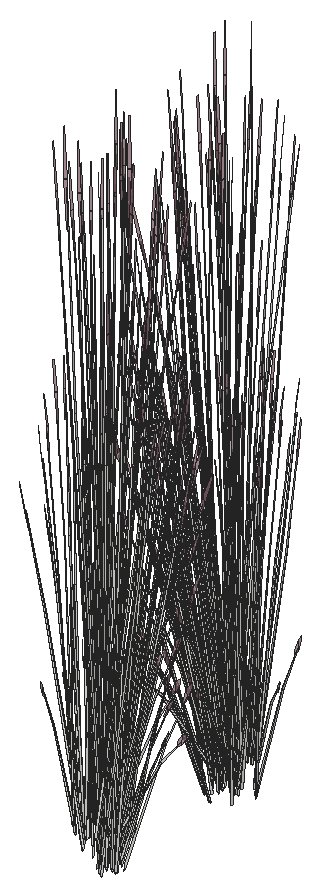
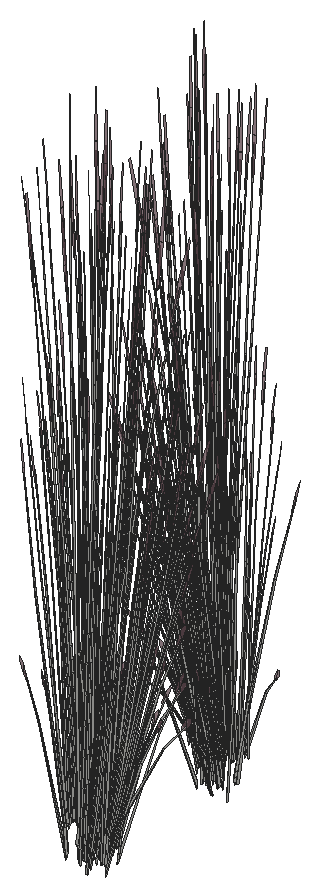
# SketchUp Ruby script. Lengths in inches.
U = 1.inch
M = Sketchup.active_model
def pt(a) = Geom::Point3d.new(a.map { |v| v * U })
def face(e, loops, mat)
  f = e.add_face(loops[0].map { |a| pt(a) })
  loops[1..].each { |l| e.add_face(l.map { |a| pt(a) }).erase! }
  f.material = f.back_material = mat if mat
  f
end
# faces: each face lists its corners as indices into pts; further lists are holes
def faces(e, pts, list, mat = nil) = list.each { |f| face(e, (f[0].is_a?(Array) ? f : [f]).map { |l| l.map { |i| pts[i] } }, mat) }
# xy, xz, yz: faces in a plane at the given z, y or x. An outline is a flat list of corners, or four numbers for a rectangle; further outlines are holes
def ring(l) = l.size == 4 ? [[l[0], l[1]], [l[2], l[1]], [l[2], l[3]], [l[0], l[3]]] : l.each_slice(2).to_a
def flat(e, list, mat, &to3) = list.each { |f| face(e, (f[0].is_a?(Array) ? f : [f]).map { |l| ring(l).map { |u, v| to3.(u, v) } }, mat) }
def xy(e, z, list, mat = nil) = flat(e, list, mat) { |x, y| [x, y, z] }
def xz(e, y, list, mat = nil) = flat(e, list, mat) { |x, z| [x, y, z] }
def yz(e, x, list, mat = nil) = flat(e, list, mat) { |y, z| [x, y, z] }
def lines(e, pts, list) = list.each { |a, b| e.add_line(pt(pts[a]), pt(pts[b])) }
# prism: a flat outline (further loops are holes) pulled along v
def prism(e, loops, v, mat = nil)
  f = face(e, loops, mat); d = Geom::Vector3d.new(v.map { |x| x * U })
  f.pushpull(f.normal.samedirection?(d) ? d.length : -d.length)
end
def box(e, o, s, mat = nil) = prism(e, [[o, [o[0] + s[0], o[1], o[2]], [o[0] + s[0], o[1] + s[1], o[2]], [o[0], o[1] + s[1], o[2]]]], [0, 0, s[2]], mat)
def at(x, y, z, deg = 0) = Geom::Transformation.translation(pt([x, y, z])) * Geom::Transformation.rotation(ORIGIN, Z_AXIS, deg.degrees)
def axes(o, x, y, z) = Geom::Transformation.new([*x, 0, *y, 0, *z, 0, *pt(o).to_a, 1])
def part(name) = M.definitions.add(name)
# library, detail: a bought-in or finely detailed component or shape, given as its bounding box
def library(name, o, s) = part(name).tap { |d| box(d.entities, o, s) }
def detail(e, o, s) = box(e.add_group.entities, o, s)
def put(e, d, t, mat = nil) = e.add_instance(d, t).tap { |i| i.material = mat if mat }
def group(e, t, mat = nil) = e.add_group.tap { |g| g.transformation = t; g.material = mat if mat }.entities
root = M.entities
M.materials.add("LightPink_Translucent").color = [144, 107, 117]
M.materials["LightPink_Translucent"].alpha = 0.75
c1 = part("blade")
p = [[2.15,0.21,22],[0,0.17,0],[0.09,0.45,0],[2.18,0.31,22],[2.29,0.31,22],[0.38,0.45,0],
  [2.48,0.24,33],[2.49,0.24,33],[2.48,0.22,33]]
faces(c1.entities,p,[[0,1,2,3],[4,5,2,3],[6,3,4,7],[8,0,3,6]])
c2 = part("seeds")
p = [[0.3,-0.1,1.38],[-0.01,-0.03,1.59],[-0.01,-0.03,0.03],[0.14,-0.07,-0.07],[0.29,-0.03,3],[0.15,0.01,3.11]]
faces(c2.entities,p,[[0,1,2,3],[1,0,4,5]],"LightPink_Translucent")
c3 = part("blade with seeds")
put(c3.entities,c1,at(0,0,0))
put(c3.entities,c2,axes([2.4,0.25,30.99],[1.5799,-0.05474,1.17369],[-0.12525,1.92788,0.29478],[-0.07173,-0.02425,1.56792]))
put(root,c3,axes([331.58,424.49,1400.18],[0.37054,-0.15823,-0.19198],[0.1302,0.45581,0.00008],[0.0409,-0.01749,1.73897]))
put(root,c3,axes([331.71,424.68,1400.47],[0.10196,-0.46348,0.17642],[0.3731,0.13116,0.35086],[-0.06445,0.00226,1.60407]))
put(root,c3,axes([331.62,423.63,1400.21],[0.24637,0.30123,0],[-0.24637,0.30123,0],[0,0,1.69266]))
put(root,c3,axes([330.22,423.0625,1401.34],[0.10032,-0.06746,1.77064],[0.0346,0.47103,0.13857],[-0.2173,0.0625,0.63284]))
put(root,c3,axes([332.29,423.5,1400.47],[-0.2773,-0.3397,0.17642],[0.27945,-0.32949,0.35086],[-0.03063,0.06937,1.60407]))
put(root,c3,axes([331.78,422.99,1400.06],[0.36714,0.07646,-0.62353],[-0.07747,0.47163,-0.16365],[0.10956,0.05715,1.37633]))
put(root,c3,axes([333.4,423.81,1400.77],[-0.21807,0.07699,1.1486],[0.10265,-0.31819,0.84392],[0.11568,0.02177,0.25299]))
put(root,c3,axes([331.07,424.73,1400.2],[-0.35581,-0.20937,0],[0.17124,-0.43505,0],[0,0,1.62707]))
put(root,c3,axes([331.36,424.17,1400.46],[-0.34464,-0.37536,-0.25192],[0.29,-0.42149,0.5513],[-0.0928,0.04391,1.68216]))
put(root,c3,axes([330.45,424.89,1400.48],[0.33032,0.23318,0.49651],[-0.19744,0.41812,0],[-0.07523,-0.05311,1.57504]))
put(root,c3,axes([331.62,423.28,1400.72],[0.17124,-0.42022,0.44739],[0.35581,0.20224,-0.21531],[0,0.09687,1.43643]))
put(root,c3,axes([333.3,425.16,1402.71],[-0.03191,-0.04083,1.77383],[0.06981,-0.43764,-0.16761],[0.12571,-0.02796,0.31391]))
put(root,c3,axes([329.14,423.38,1402.72],[-0.05763,0.06055,1.74944],[0.0049,0.44239,-0.27667],[-0.13211,0.05753,0.14031]))
put(root,c3,axes([331.55,423.52,1400.29],[0,0.53934,-0.05637],[-0.44133,0,0],[0,0.01695,1.79368]))
put(root,c3,axes([329.53,423.32,1402.68],[-0.09562,0.42421,-0.51099],[-0.32782,-0.1454,-0.3958],[-0.13199,0.0389,0.97773]))
put(root,c3,axes([329.51,422.96,1403.03],[0.17758,0.42229,-0.1216],[-0.31518,0.20752,-0.67495],[-0.13282,0.05572,1.02557]))
put(root,c3,axes([331.58,423.14,1400.21],[0.21202,0.39143,-0.44739],[-0.32115,0.27564,0.21531],[0.06861,0.04843,1.43643]))
put(root,c3,axes([333.02,424.79,1401.93],[-0.06755,-0.39203,-0.03492],[0.31928,-0.09013,-0.15832],[0.06667,0.02485,0.52218]))
put(root,c3,axes([330.26,425.13,1400.375],[-0.22066,0.46731,0],[-0.36918,-0.26061,-0.51607],[-0.08408,-0.05936,1.63711]))
put(root,c3,axes([332.19,424.78,1403.03],[0.0189,-0.47427,-0.1216],[0.35781,0.01296,-0.67495],[0.13781,0.03295,1.02557]))
put(root,c3,axes([332.52,423.51,1400.48],[0,-0.46636,0.49651],[0.39487,0,0],[0,0.10622,1.57504]))
put(root,c3,axes([331.53,423.86,1400.72],[0.38326,-0.02879,0.44739],[0.03466,0.47788,-0.21531],[-0.06861,0.04843,1.43643]))
put(root,c3,axes([331.77,423.375,1400.62],[0.32884,-0.136,0.1448],[0.11516,0.38837,-0.41347],[0,0.08547,1.26744]))
put(root,c3,axes([332.14,424.59,1403.05],[-0.20082,-0.29199,0.35414],[0.2293,-0.2764,-0.4572],[0.1165,0.04206,0.87481]))
put(root,c3,axes([331.1875,424.09,1400.21],[-0.38326,0.02879,-0.44739],[-0.03466,-0.47788,0.21531],[-0.06861,0.04843,1.43643]))
put(root,c3,axes([332.99,424.32,1400.59],[-0.085,-0.1147,1.43002],[0.1106,-0.37943,-0.30754],[0.17198,0.0514,0.61141]))
put(root,c3,axes([331.47,424.74,1400.2],[0.35581,0.20937,0],[-0.17124,0.43505,0],[0,0,1.74954]))
put(root,c3,axes([332.5,424.49,1402.72],[0.07571,-0.00789,1.74944],[0.20767,-0.36231,-0.27667],[0.13467,0.04783,0.14031]))
put(root,c3,axes([331.61,425.2,1400.19],[-0.21791,-0.46895,-0.05142],[0.36918,-0.26061,0.51607],[-0.09097,0.04465,1.6363]))
put(root,c3,axes([331.53,424.07,1400.62],[0.26075,0.2802,0.1448],[-0.2175,0.31612,-0.41347],[-0.06054,0.04274,1.26744]))
put(root,c3,axes([329.47,424.14,1402.73],[-0.08753,-0.42921,0.48003],[0.34336,-0.07449,0.3958],[-0.1012,0.10094,0.9933]))
put(root,c3,axes([329.41,424.06,1402.73],[-0.2423,-0.19613,0.0643],[0.14107,-0.2793,0.50621],[-0.07768,0.0903,0.77189]))
put(root,c3,axes([329.52,423.54,1401.875],[0.12246,-0.09864,1.71376],[0.1031,0.45582,0.13857],[-0.19225,0.10302,0.73262]))
put(root,c3,axes([332.21,424.55,1402.98],[0.35281,0.01123,-0.71045],[-0.0237,0.47284,0.08574],[0.14947,0.0499,1.00501]))
put(root,c3,axes([331.8125,424.93,1400.48],[0.33032,-0.23318,0.49651],[0.19744,0.41812,0],[-0.07523,0.05311,1.57504]))
put(root,c3,axes([331.34,424.5625,1400.29],[0.15345,0.53576,-0.06012],[-0.43845,0.18773,0],[0.00536,0.01871,1.72173]))
put(root,c3,axes([331.51,425.14,1400.03],[-0.32928,-0.11539,-0.30978],[0.08291,-0.40636,0.30978],[-0.06638,0.04686,1.38974]))
put(root,c3,axes([329.14,424.32,1400.59],[0.12266,0.03828,1.43002],[0.07906,0.39104,-0.30754],[-0.16661,0.0732,0.61141]))
put(root,c3,axes([329.6875,424,1403.05],[0.30722,-0.06665,0.35414],[0.08112,0.381,-0.4572],[-0.08804,0.10234,0.87481]))
put(root,c3,axes([332.78,423.59,1400.375],[0.44133,0,0],[0,0.52122,-0.51607],[0,0.11871,1.63711]))
put(root,c3,axes([328.5,423.83,1402.71],[0.04504,0.01251,1.77383],[0.13934,0.41205,-0.16761],[-0.0922,0.10815,0.31391]))
put(root,c3,axes([332.61,423.86,1400.2],[-0.44111,-0.00373,-0.04976],[0,-0.52122,0.49943],[-0.01386,0.11865,1.58352]))
put(root,c3,axes([331.65,423.4,1400.67],[0.39748,0.22252,-0.29095],[-0.19139,0.46966,-0.50002],[0.01249,0.11531,1.59708]))
put(root,c3,axes([328.88,425.14,1400.77],[0.14709,-0.21136,1.1486],[0.05804,0.3346,0.84392],[-0.1063,0.05991,0.25299]))
put(root,c3,axes([332.42,424.75,1402.53],[0.20082,0.29199,-0.35414],[-0.2293,0.2764,0.4572],[0.1165,0.04206,0.87481]))
put(root,c3,axes([332.52,423.93,1400.03],[-0.24637,0.29097,-0.30978],[-0.24637,-0.29097,0.30978],[0,0.09372,1.38974]))
put(root,c3,axes([331.46,423.96,1400.67],[0.04113,0.53214,-0.29095],[-0.42835,0.03218,-0.50002],[-0.07543,0.07088,1.59708]))
put(root,c3,axes([332.32,424.86,1402.73],[-0.01777,0.35463,0.0643],[-0.26836,-0.00972,0.50621],[0.1028,0.03711,0.77189]))
put(root,c3,axes([331.61,423.75,1400.21],[-0.17124,0.42022,-0.44739],[-0.35581,-0.20224,0.21531],[0,0.09687,1.43643]))
put(root,c3,axes([329.43,424.22,1402.53],[-0.30722,0.06665,-0.35414],[-0.08112,-0.381,0.4572],[-0.08804,0.10234,0.87481]))
put(root,c3,axes([332.34,424.74,1402.73],[-0.26024,0.30729,0.48003],[-0.22444,-0.32634,0.3958],[0.1221,0.05668,0.9933]))
put(root,c3,axes([328.99,425.08,1403.65],[0.31145,0.12449,-0.06488],[-0.0958,0.38314,-0.29416],[-0.05094,0.05817,0.97024]))
put(root,c3,axes([331.2,424.37,1400.06],[-0.23773,0.35053,-0.62353],[-0.29532,-0.31785,-0.16365],[-0.09526,0.08744,1.37633]))
put(root,c3,axes([331.52,425.1,1403.05],[-0.05451,-0.37564,0.35414],[0.31161,-0.09919,-0.4572],[0.0837,0.10765,0.87481]))
put(root,c3,axes([331.62,424.96,1400.33],[0.44186,0.15158,0.30756],[-0.11054,0.54181,-0.36492],[-0.07313,0.06781,1.64885]))
put(root,c3,axes([331.59,425.32,1400.02],[-0.33032,0.23318,-0.49651],[-0.19744,-0.41812,0],[-0.07523,0.05311,1.57504]))
put(root,c3,axes([332.6875,423.94,1400.02],[0,0.46636,-0.49651],[-0.39487,0,0],[0,0.10622,1.57504]))
put(root,c3,axes([331.7,424,1401.875],[-0.1311,-0.08035,1.71376],[0.27131,-0.33708,0.13857],[0.16909,0.15206,0.73262]))
put(root,c3,axes([331.72,422.9375,1402.47],[-0.30498,-0.24231,1.38283],[0.32203,-0.37727,0.59665],[0.0984,0.22736,1.33663]))
put(root,c3,axes([329.53,423.96,1403.03],[0.32648,0.25715,-0.1216],[-0.18809,0.3724,-0.67495],[-0.09224,0.12945,1.02557]))
put(root,c3,axes([332.18,424.91,1400.77],[-0.19872,-0.13409,1.1486],[0.2566,-0.13625,0.84392],[0.06921,0.11541,0.25299]))
put(root,c3,axes([331.49,425.29,1403.03],[0.21031,-0.39918,-0.1216],[0.30457,0.22997,-0.67495],[0.10587,0.11278,1.02557]))
put(root,c3,axes([329.97,423.85,1401.875],[0.08815,-0.14329,1.71376],[0.22258,0.38678,0.13857],[-0.15267,0.17614,0.73262]))
put(root,c3,axes([329.6875,424.27,1402.68],[0.09067,0.42583,-0.51099],[-0.34336,0.07449,-0.3958],[-0.0984,0.11438,0.97773]))
put(root,c3,axes([330.1,424.76,1403.05],[0.23881,-0.24554,0.35414],[0.22606,0.28036,-0.4572],[-0.0344,0.14245,0.87481]))
put(root,c3,axes([331.89,425.25,1400.375],[0.22066,0.46731,0],[-0.36918,0.26061,-0.51607],[-0.08408,0.05936,1.63711]))
put(root,c3,axes([331.21,425.625,1402.71],[0.00104,-0.05646,1.77383],[0.30246,-0.2491,-0.16761],[0.10506,0.08891,0.31391]))
put(root,c3,axes([332.24,425.41,1399.49],[0.02571,-0.06733,1.76342],[0.32373,-0.19829,-0.26939],[0.09815,0.10263,0.30037]))
put(root,c3,axes([331.7,423.4,1400.84],[-0.00964,-0.43909,1.41272],[0.43635,0.11382,0.59816],[-0.1032,0.24027,1.3335]))
put(root,c3,axes([331.8125,423.88,1400.09],[0.12941,0.42699,-0.69212],[-0.37279,0.15378,-0.18165],[0.0143,0.14459,1.52773]))
put(root,c3,axes([329.88,424.98,1402.73],[-0.29004,-0.02173,0.0643],[0.00795,-0.32812,0.50621],[-0.03035,0.12569,0.77189]))
put(root,c3,axes([329.27,425.35,1399.49],[0.04734,0.04659,1.76342],[0.08027,0.4317,-0.26939],[-0.10492,0.09206,0.30037]))
put(root,c3,axes([329.98,425.01,1402.73],[-0.25132,-0.3182,0.48003],[0.2669,-0.27442,0.3958],[-0.04636,0.14929,0.9933]))
put(root,c3,axes([331.74,425.1,1402.68],[0.34827,-0.11086,-0.51099],[0.06092,0.41983,-0.3958],[0.09354,0.12031,0.97773]))
put(root,c3,axes([330.77,425.16,1403.05],[0.1064,-0.35863,0.35414],[0.31043,0.1046,-0.4572],[0.02846,0.14439,0.87481]))
put(root,c3,axes([332.22,425.52,1400.67],[-0.22633,-0.01463,1.0506],[0.14947,-0.31064,0.58006],[0.08941,0.11036,0.8241]))
put(root,c3,axes([331.56,425.44,1402.73],[-0.16041,0.29625,0.0643],[-0.22843,-0.17248,0.50621],[0.07385,0.09498,0.77189]))
put(root,c3,axes([331.1875,426.4375,1403.65],[0.2439,-0.26754,-0.06488],[0.22348,0.29302,-0.29416],[0.01573,0.08303,0.97024]))
put(root,c3,axes([331.63,425.36,1402.73],[-0.35104,0.10702,0.48003],[-0.06092,-0.41983,0.3958],[0.08256,0.12373,0.9933]))
put(root,c3,axes([329.9,424.2,1401.875],[0.06572,-0.16029,1.71376],[0.27569,0.33172,0.13857],[-0.12437,0.20675,0.73262]))
put(root,c3,axes([331.48,424.77,1400.59],[0.00623,-0.15459,1.43002],[0.29764,-0.17268,-0.30754],[0.09188,0.18503,0.61141]))
put(root,c3,axes([330.67,425.48,1402.73],[-0.26007,0.1585,0.0643],[-0.12729,-0.28902,0.50621],[0.02512,0.1274,0.77189]))
put(root,c3,axes([329.98,425.1,1402.53],[-0.23881,0.24554,-0.35414],[-0.22606,-0.28036,0.4572],[-0.0344,0.14245,0.87481]))
put(root,c3,axes([329.15,425.03,1402.72],[-0.00877,0.09229,1.74944],[0.24897,0.32105,-0.27667],[-0.06518,0.15182,0.14031]))
put(root,c3,axes([329.95,424.82,1403.4],[0.3879,0.02311,-0.13498],[-0.0106,0.43749,-0.74919],[-0.02694,0.1685,1.13838]))
put(root,c3,axes([330.67,425.31,1403.03],[0.34538,-0.21713,-0.1216],[0.16972,0.38536,-0.67495],[0.04557,0.16239,1.02557]))
put(root,c3,axes([330.77,425.45,1403.0625],[-0.34777,-0.12192,0.53283],[0.11892,-0.40083,0.43934],[0.0209,0.15763,1.10256]))
put(root,c3,axes([330.13,426.06,1400.77],[-0.00913,-0.2773,1.1486],[0.22824,0.19778,0.84392],[-0.04489,0.13217,0.25299]))
put(root,c3,axes([330.73,425.39,1399.49],[0.05712,-0.02538,1.76342],[0.34359,0.13968,-0.26939],[0.01005,0.15742,0.30037]))
put(root,c3,axes([330.21,424.99,1403],[0.25266,0.31335,-0.5672],[-0.2669,0.27442,-0.43934],[-0.03844,0.15921,1.08528]))
put(root,c3,axes([329.9375,425.46,1400.82],[0.32063,-0.08258,0.06507],[0.07371,0.33271,-0.86304],[-0.02033,0.16842,0.7736]))
put(root,c3,axes([330.96,425.29,1402.68],[0.34695,0.11691,-0.51099],[-0.11892,0.40083,-0.3958],[0.03181,0.16138,0.97773]))
put(root,c3,axes([331.16,424.46,1401.875],[-0.08068,-0.14973,1.71376],[0.3728,-0.12606,0.13857],[0.08426,0.23506,0.73262]))
put(root,c3,axes([330.8,425.54,1402.53],[-0.1064,0.35863,-0.35414],[-0.31043,-0.1046,0.4572],[0.02846,0.14439,0.87481]))
put(root,c3,axes([330.13,424.84,1403.34],[-0.00918,0.43138,-0.7886],[-0.38672,-0.02897,0.09517],[-0.04081,0.18275,1.11556]))
put(root,c3,axes([329.125,425.98,1402.71],[0.04004,-0.02816,1.77383],[0.33095,0.18728,-0.16761],[-0.00778,0.15594,0.31391]))
put(root,c3,axes([330.5,424.54,1401.875],[-0.00864,-0.17899,1.71376],[0.37441,0.11874,0.13857],[-0.02316,0.25508,0.73262]))
put(root,c3,axes([330.84,425.22,1402.98],[0.16845,0.3792,-0.71045],[-0.34676,0.21133,0.08574],[0.03939,0.18322,1.00501]))
put(root,c3,axes([329.86,425.8125,1400.59],[0.11138,-0.07357,1.43002],[0.27499,0.22183,-0.30754],[-0.08185,0.19194,0.61141]))
put(root,c3,axes([330.58,426.17,1402.72],[0.04474,0.0751,1.74944],[0.36104,0.0295,-0.27667],[0.03631,0.16562,0.14031]))
put(root,c3,axes([330.01,425.45,1401.36],[0.00775,-0.24075,1.54345],[0.34877,0.12716,0.21329],[-0.03022,0.25658,0.72882]))
put(root,c3,axes([330.27,437.97,1401.875],[0.08068,0.14973,1.71376],[-0.3728,0.12606,0.13857],[-0.08426,-0.23506,0.73262]))
put(root,c3,axes([330.89,436.98,1402.72],[-0.05398,-0.06539,1.74944],[-0.36026,0.04145,-0.27667],[-0.0575,-0.15639,0.14031]))
put(root,c3,axes([331.72,437.76,1400.59],[-0.10032,0.0944,1.43002],[-0.30046,-0.16522,-0.30754],[0.05569,-0.20547,0.61141]))
put(root,c3,axes([331.27,438.09,1402.98],[-0.16845,-0.3792,-0.71045],[0.34676,-0.21133,0.08574],[-0.03939,-0.18322,1.00501]))
put(root,c3,axes([330.17,437.58,1400.59],[-0.02137,0.15256,1.43002],[-0.31245,0.12771,-0.30754],[-0.07303,-0.19719,0.61141]))
put(root,c3,axes([330.98,437.24,1399.49],[-0.0592,0.0168,1.76342],[-0.32738,-0.18913,-0.26939],[0.00549,-0.15776,0.30037]))
put(root,c3,axes([331.97,438.46,1402.98],[0.00918,-0.43138,-0.71045],[0.38672,0.02897,0.08574],[0.04081,-0.18275,1.00501]))
put(root,c3,axes([332.51,437.78,1402.72],[-0.00341,-0.09282,1.74944],[-0.28775,-0.26825,-0.27667],[0.04449,-0.16261,0.14031]))
put(root,c3,axes([331.3,437.76,1402.53],[0.1064,-0.35863,-0.35414],[0.31043,0.1046,0.4572],[-0.02846,-0.14439,0.87481]))
put(root,c3,axes([331.53,438.24,1401.875],[-0.06572,0.16029,1.71376],[-0.27569,-0.33172,0.13857],[0.12437,-0.20675,0.73262]))
put(root,c3,axes([332.43,437.45,1402.71],[-0.03584,0.03562,1.77383],[-0.35118,-0.12018,-0.16761],[-0.01271,-0.15545,0.31391]))
put(root,c3,axes([331.14,438.01,1402.68],[-0.34695,-0.11691,-0.51099],[0.11892,-0.40083,-0.3958],[-0.03181,-0.16138,0.97773]))
put(root,c3,axes([331.35,437.01,1400.77],[0.04528,0.27194,1.1486],[-0.25117,-0.15062,0.84392],[0.02703,-0.13924,0.25299]))
put(root,c3,axes([331.89,438.3125,1402.68],[-0.25266,-0.31335,-0.51099],[0.2669,-0.27442,-0.3958],[0.03844,-0.15921,0.97773]))
put(root,c3,axes([330.52,436.77,1402.71],[-0.00658,0.0559,1.77383],[-0.32474,0.20287,-0.16761],[-0.09556,-0.1037,0.31391]))
put(root,c3,axes([330.45,437.76,1403.09],[0.39316,-0.11987,0.53763],[0.06823,0.47021,0.4433],[-0.09247,-0.13858,1.11249]))
put(root,c3,axes([331.34,437.85,1402.73],[0.34777,0.12192,0.48003],[-0.11892,0.40083,0.3958],[-0.0209,-0.15763,0.9933]))
put(root,c3,axes([331.4375,437.99,1403.03],[-0.34538,0.21713,-0.1216],[-0.16972,-0.38536,-0.67495],[-0.04557,-0.16239,1.02557]))
put(root,c3,axes([332.15,438.48,1403.03],[-0.3879,-0.02311,-0.1216],[0.0106,-0.43749,-0.67495],[0.02694,-0.1685,1.02557]))
put(root,c3,axes([332.13,438.2,1402.53],[0.23881,-0.24554,-0.35414],[0.22606,0.28036,0.4572],[0.0344,-0.14245,0.87481]))
put(root,c3,axes([330.0625,437.33,1400.77],[0.18411,0.16231,1.1486],[-0.26813,0.09757,0.84392],[-0.05737,-0.12474,0.25299]))
put(root,c3,axes([331.43,437.82,1402.73],[0.26007,-0.1585,0.0643],[0.12729,0.28902,0.50621],[-0.02512,-0.1274,0.77189]))
put(root,c3,axes([330.51,438.19,1402.98],[-0.30095,-0.22541,-0.71045],[0.21388,-0.395,0.08574],[-0.10904,-0.13459,1.00501]))
put(root,c3,axes([330.4,437.9,1402.53],[-0.05451,-0.37564,-0.35414],[0.31161,-0.09919,0.4572],[-0.0837,-0.10765,0.87481]))
put(root,c3,axes([330.54,437.86,1402.73],[0.16041,-0.29625,0.0643],[0.22843,0.17248,0.50621],[-0.07385,-0.09498,0.77189]))
put(root,c3,axes([329.92,437.82,1399.49],[-0.03419,0.06144,1.76342],[-0.3455,0.13246,-0.26939],[-0.08346,-0.12049,0.30037]))
put(root,c3,axes([330.49,439.51,1400.1],[-0.14494,-0.47823,-0.69835],[0.41752,-0.17223,-0.18329],[-0.01602,-0.16194,1.54149]))
put(root,c3,axes([329.73,438.44,1401.875],[0.1311,0.08035,1.71376],[-0.27131,0.33708,0.13857],[-0.16909,-0.15206,0.73262]))
put(root,c3,axes([332.43,438.05,1399.49],[-0.05283,-0.03674,1.76342],[-0.13569,-0.41045,-0.26939],[0.09154,-0.11138,0.30037]))
put(root,c3,axes([331.33,438.14,1403.05],[-0.1064,0.35863,0.35414],[-0.31043,-0.1046,-0.4572],[-0.02846,-0.14439,0.87481]))
put(root,c3,axes([330.37,438.2,1402.68],[-0.34827,0.11086,-0.51099],[-0.06092,-0.41983,-0.3958],[-0.09354,-0.12031,0.97773]))
put(root,c3,axes([332.125,438.29,1402.73],[0.25132,0.3182,0.48003],[-0.2669,0.27442,0.3958],[0.04636,-0.14929,0.9933]))
put(root,c3,axes([330.61,437.83,1403.43],[-0.23555,0.44708,-0.13619],[-0.34112,-0.25757,-0.75594],[-0.11858,-0.12631,1.14864]))
put(root,c3,axes([332.22,438.32,1402.73],[0.29004,0.02173,0.0643],[-0.00795,0.32812,0.50621],[0.03035,-0.12569,0.77189]))
put(root,c3,axes([332,438.55,1403.05],[-0.23881,0.24554,0.35414],[-0.22606,-0.28036,-0.4572],[0.0344,-0.14245,0.87481]))
put(root,c3,axes([332.42,439.21,1402.98],[0.18436,-0.36797,-0.71045],[0.32306,0.26151,0.08574],[0.11008,-0.13332,1.00501]))
put(root,c3,axes([330.43,438.14,1400.375],[-0.22066,-0.46731,0],[0.36918,-0.26061,-0.51607],[0.08408,-0.05936,1.63711]))
put(root,c3,axes([332.41,439.03,1402.68],[-0.09067,-0.42583,-0.51099],[0.34336,-0.07449,-0.3958],[0.0984,-0.11438,0.97773]))
put(root,c3,axes([330.92,437.57,1400.13],[-0.2439,0.26754,-0.03893],[-0.22348,-0.29302,-0.17649],[-0.01573,-0.08303,0.58215]))
put(root,c3,axes([329.71,437.7,1402.72],[-0.07594,-0.00329,1.74944],[-0.24177,0.32918,-0.27667],[-0.129,-0.06726,0.14031]))
put(root,c3,axes([332.58,439.34,1403.03],[-0.32648,-0.25715,-0.1216],[0.18809,-0.3724,-0.67495],[0.09224,-0.12945,1.02557]))
put(root,c3,axes([331.23,440.74,1401.33],[0.305,0.18805,1.51261],[-0.29879,0.40513,0.59816],[-0.13384,-0.24012,1.26806]))
put(root,c3,axes([330.59,438.2,1403.05],[0.05451,0.37564,0.35414],[-0.31161,0.09919,-0.4572],[-0.0837,-0.10765,0.87481]))
put(root,c3,axes([329.63,439.44,1400.02],[0,-0.46636,-0.49651],[0.39487,0,0],[0,-0.10622,1.57504]))
put(root,c3,axes([330.73,438.0625,1400.02],[0.33032,-0.23318,-0.49651],[0.19744,0.41812,0],[0.07523,-0.05311,1.57504]))
put(root,c3,axes([332.69,438.87,1400.59],[-0.12609,-0.01381,1.43002],[-0.12917,-0.37055,-0.30754],[0.1549,-0.10482,0.61141]))
put(root,c3,axes([329.65,438.45,1403.09],[0.29147,-0.34417,0.53763],[0.25138,0.3655,0.4433],[-0.13675,-0.06349,1.11249]))
put(root,c3,axes([333.38,439.23,1402.71],[-0.0461,-0.00354,1.77383],[-0.19143,-0.37951,-0.16761],[0.07688,-0.12478,0.31391]))
put(root,c3,axes([331.12,439.02,1400.06],[0.23773,-0.35053,-0.62353],[0.29532,0.31785,-0.16365],[0.09526,-0.08744,1.37633]))
put(root,c3,axes([332.84,438.1875,1400.77],[-0.11756,0.2374,1.1486],[-0.10105,-0.31895,0.84392],[0.09709,-0.07992,0.25299]))
put(root,c3,axes([332.67,439.08,1402.53],[0.30722,-0.06665,-0.35414],[0.08112,0.381,0.4572],[0.08804,-0.10234,0.87481]))
put(root,c3,axes([329.78,438.44,1402.73],[0.01777,-0.35463,0.0643],[0.26836,0.00972,0.50621],[-0.1028,-0.03711,0.77189]))
put(root,c3,axes([330.71,439.63,1400.21],[0.17124,-0.42022,-0.44739],[0.35581,0.20224,0.21531],[0,-0.09687,1.43643]))
put(root,c3,axes([329.68,438.56,1402.53],[-0.20082,-0.29199,-0.35414],[0.2293,-0.2764,0.4572],[-0.1165,-0.04206,0.87481]))
put(root,c3,axes([330.86,439.43,1400.67],[-0.04113,-0.53214,-0.29095],[0.42835,-0.03218,-0.50002],[0.07543,-0.07088,1.59708]))
put(root,c3,axes([329.8,439.45,1400.03],[0.24637,-0.29097,-0.30978],[0.24637,0.29097,0.30978],[0,-0.09372,1.38974]))
put(root,c3,axes([329.7,438.06,1400.13],[-0.10181,0.3808,-0.03893],[-0.31336,-0.11714,-0.17649],[-0.04758,-0.06228,0.58215]))
put(root,c3,axes([332.42,439.3,1403.05],[-0.30722,0.06665,0.35414],[-0.08112,-0.381,-0.4572],[0.08804,-0.10234,0.87481]))
put(root,c3,axes([330.67,439.98,1400.67],[-0.39748,-0.22252,-0.29095],[0.19139,-0.46966,-0.50002],[-0.01249,-0.11531,1.59708]))
put(root,c3,axes([329.53,439.8,1400.375],[-0.44133,0,0],[0,-0.52122,-0.51607],[0,-0.11871,1.63711]))
put(root,c3,axes([329.61,438.87,1400.59],[0.06891,0.12984,1.43002],[-0.15879,0.35293,-0.30754],[-0.16304,-0.08436,0.61141]))
put(root,c3,axes([330.81,438.25,1400.03],[0.32928,0.11539,-0.30978],[-0.08291,0.40636,0.30978],[0.06638,-0.04686,1.38974]))
put(root,c3,axes([329.89,438.75,1402.98],[-0.35281,-0.01123,-0.71045],[0.0237,-0.47284,0.08574],[-0.14947,-0.0499,1.00501]))
put(root,c3,axes([332.7,439.24,1402.73],[0.2423,0.19613,0.0643],[-0.14107,0.2793,0.50621],[0.07768,-0.0903,0.77189]))
put(root,c3,axes([332.63,439.16,1402.73],[0.08753,0.42921,0.48003],[-0.34336,0.07449,0.3958],[0.1012,-0.10094,0.9933]))
put(root,c3,axes([333.55,439.68,1402.72],[0.04898,-0.07104,1.74944],[-0.06269,-0.43574,-0.27667],[0.12289,-0.08262,0.14031]))
put(root,c3,axes([329.875,439.66,1400.33],[-0.32829,0.39208,0.30756],[-0.32849,-0.38796,-0.36492],[-0.01146,-0.11134,1.64885]))
put(root,c3,axes([329.42,437.98,1402.71],[0.02617,0.04654,1.77383],[-0.12614,0.41836,-0.16761],[-0.12775,0.00303,0.31391]))
put(root,c3,axes([330.92,439.84,1400.43],[0.39767,0.22603,0.24065],[-0.19139,0.46966,0.50002],[0,-0.10827,1.60543]))
put(root,c3,axes([330.77,440.48,1400.4375],[0.09355,-0.55261,-0.23429],[0.44354,0.09633,0.51271],[-0.0775,-0.07631,1.5644]))
put(root,c3,axes([329.78,438.85,1402.68],[-0.25628,0.30892,-0.51099],[-0.22444,-0.32634,-0.3958],[-0.13021,-0.047,0.97773]))
put(root,c3,axes([329.97,438.71,1403.05],[0.20082,0.29199,0.35414],[-0.2293,0.2764,-0.4572],[-0.1165,-0.04206,0.87481]))
put(root,c3,axes([329.2,439.26,1400.77],[0.22533,-0.03337,1.1486],[-0.14293,0.29403,0.84392],[-0.11135,-0.04411,0.25299]))
put(root,c3,axes([330.79,439.53,1400.72],[-0.38326,0.02879,0.44739],[-0.03466,-0.47788,-0.21531],[0.06861,-0.04843,1.43643]))
put(root,c3,axes([329.91,438.52,1403.03],[-0.0189,0.47427,-0.1216],[-0.35781,-0.01296,-0.67495],[-0.13781,-0.03295,1.02557]))
put(root,c3,axes([329.8,439.875,1400.48],[0,0.46636,0.49651],[-0.39487,0,0],[0,-0.10622,1.57504]))
put(root,c3,axes([332.59,440.34,1403.03],[-0.17758,-0.42229,-0.1216],[0.31518,-0.20752,-0.67495],[0.13282,-0.05572,1.02557]))
put(root,c3,axes([332.57,439.98,1402.68],[0.09562,-0.42421,-0.51099],[0.32782,0.1454,-0.3958],[0.13199,-0.0389,0.97773]))
put(root,c3,axes([332.06,438.25,1400.375],[0.22066,-0.46731,0],[0.36918,0.26061,-0.51607],[0.08408,0.05936,1.63711]))
put(root,c3,axes([329.46,439.18,1401.875],[0.14639,-0.01056,1.71376],[-0.09712,0.45778,0.13857],[-0.20862,-0.02831,0.73262]))
put(root,c3,axes([330.73,440.25,1400.21],[-0.21202,-0.39143,-0.44739],[0.32115,-0.27564,0.21531],[-0.06861,-0.04843,1.43643]))
put(root,c3,axes([330.78,439.7,1400.36],[0.15345,0.52148,0.45755],[-0.43845,0.18134,0.17955],[0.00536,-0.09582,1.58856]))
put(root,c3,axes([332.92,440.1,1399.98],[-0.22732,0.05597,1.41583],[-0.03618,-0.44548,0.08104],[0.15921,-0.06743,0.80566]))
put(root,c3,axes([333.34,439.71,1400.26],[-0.21881,-0.29821,-0.06488],[0.23965,-0.27324,-0.29416],[0.0679,-0.01924,0.97024]))
put(root,c3,axes([330.7,440.11,1400.72],[-0.17124,0.42022,0.44739],[-0.35581,-0.20224,-0.21531],[0,-0.09687,1.43643]))
put(root,c3,axes([331.33,439.74,1400.21],[0,-0.53961,0],[0.44133,0,0],[0,0,1.79456]))
put(root,c3,axes([331.87,438.5,1400.48],[-0.33032,-0.23318,0.49651],[0.19744,-0.41812,0],[0.07523,0.05311,1.57504]))
put(root,c3,axes([332.51,440.13,1402.98],[0.31014,-0.20596,-0.71045],[0.17284,0.42397,0.08574],[0.14985,-0.04816,1.00501]))
put(root,c3,axes([330.54,440.4,1400.06],[-0.36714,-0.07646,-0.62353],[0.07747,-0.47163,-0.16365],[-0.10956,-0.05715,1.37633]))
put(root,c3,axes([331.12,439.4,1400.36],[-0.29264,0.42323,0.45755],[-0.34767,-0.3736,0.17955],[0.07055,-0.04224,1.58856]))
put(root,c3,axes([331.44,440.16,1400.3],[-0.32829,-0.4014,-0.06131],[0.32849,-0.40164,0],[-0.01146,-0.01402,1.75571]))
put(root,c3,axes([330.61,438.71,1400.47],[-0.10196,0.46348,0.17642],[-0.3731,-0.13116,0.35086],[0.06445,-0.00226,1.60407]))
put(root,c3,axes([332.47,440.22,1403.05],[-0.29332,-0.1301,0.35414],[0.08555,-0.37955,-0.4572],[0.11809,-0.0348,0.87481]))
put(root,c3,axes([329.4,439.52,1402.73],[0.09971,-0.42522,0.48003],[0.32782,0.1454,0.3958],[-0.12892,0.02555,0.9933]))
put(root,c3,axes([330.46,439.08,1399.59],[-0.3474,0.18671,1.28929],[-0.11057,-0.53572,0.50096],[0.21332,0.00891,1.46642]))
put(root,c3,axes([331.39,439.22,1400.62],[0.06809,-0.4162,0.1448],[0.33266,0.07225,-0.41347],[0.06054,0.04274,1.26744]))
put(root,c3,axes([329.37,439.41,1402.73],[-0.12963,-0.31798,0.0643],[0.23638,-0.15564,0.50621],[-0.1042,0.03071,0.77189]))
put(root,c3,axes([330.82,440.21,1400.36],[0.44609,0.09826,0.45755],[-0.09078,0.55493,0.17955],[-0.06519,-0.05359,1.58856]))
put(root,c3,axes([333.17,439.81,1399.49],[-0.01845,-0.0708,1.76342],[0.12793,-0.41416,-0.26939],[0.12905,-0.00596,0.30037]))
put(root,c3,axes([329.36,439.74,1399.49],[0.00895,0.0735,1.76342],[-0.18044,0.38382,-0.26939],[-0.12817,-0.01935,0.30037]))
put(root,c3,axes([331.25,439.33,1400.72],[-0.21202,-0.39143,0.44739],[0.32115,-0.27564,-0.21531],[0.06861,0.04843,1.43643]))
put(root,c3,axes([330.15,441.12,1400.03],[-0.08291,-0.40636,-0.30978],[0.32928,-0.11539,0.30978],[-0.06638,-0.04686,1.38974]))
put(root,c3,axes([330.58,441.1,1400.47],[0.37926,-0.12378,0.17642],[0.09365,0.46065,0.35086],[-0.03382,-0.06712,1.60407]))
put(root,c3,axes([331.36,439.36,1400.67],[0.35635,-0.30962,-0.29095],[0.23697,0.43749,-0.50002],[0.08792,0.04443,1.59708]))
put(root,c3,axes([332.78,440.17,1402.53],[0.29332,0.1301,-0.35414],[-0.08555,0.37955,0.4572],[0.11809,-0.0348,0.87481]))
put(root,c3,axes([330.0625,441.3,1400.02],[-0.33032,-0.23318,-0.49651],[0.19744,-0.41812,0],[-0.07523,-0.05311,1.57504]))
put(root,c3,axes([332.26,438.53,1400.02],[0.33032,0.23318,-0.49651],[-0.19744,0.41812,0],[0.07523,0.05311,1.57504]))
put(root,c3,axes([329.33,439.57,1402.53],[-0.29332,-0.1301,-0.35414],[0.08555,-0.37955,0.4572],[-0.11809,0.0348,0.87481]))
put(root,c3,axes([331.63,439.86,1400.21],[0.39487,0,0],[0,0.48281,0],[0,0,1.78407]))
